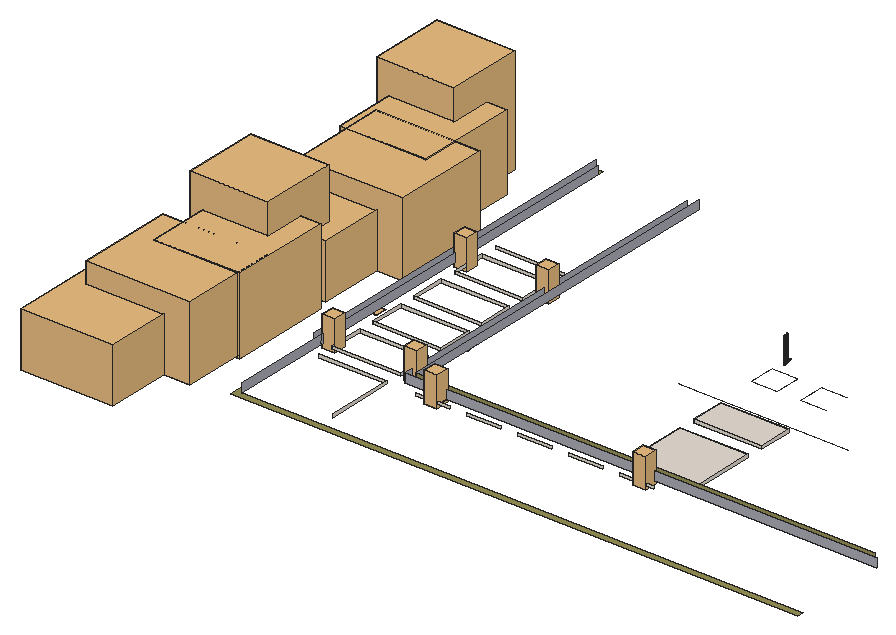
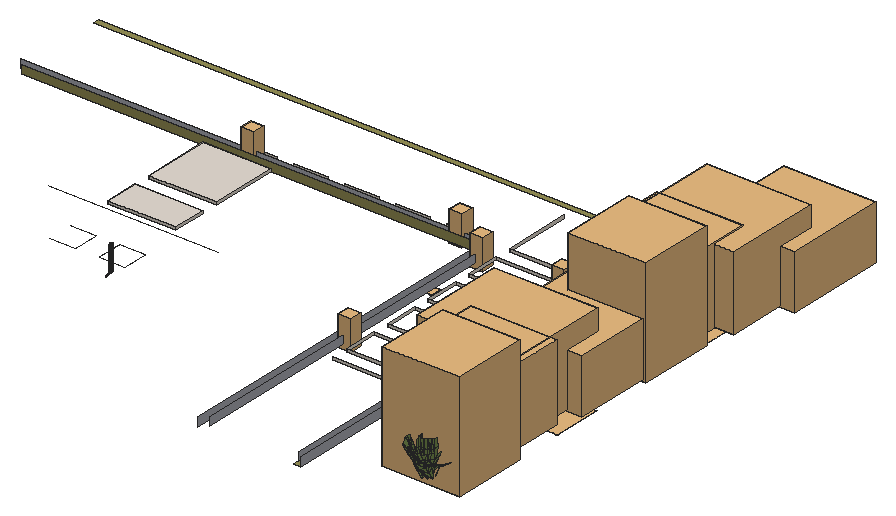
# SketchUp Ruby script. Lengths in inches.
U = 1.inch
M = Sketchup.active_model
def pt(a) = Geom::Point3d.new(a.map { |v| v * U })
def face(e, loops, mat)
  f = e.add_face(loops[0].map { |a| pt(a) })
  loops[1..].each { |l| e.add_face(l.map { |a| pt(a) }).erase! }
  f.material = f.back_material = mat if mat
  f
end
# faces: each face lists its corners as indices into pts; further lists are holes
def faces(e, pts, list, mat = nil) = list.each { |f| face(e, (f[0].is_a?(Array) ? f : [f]).map { |l| l.map { |i| pts[i] } }, mat) }
# xy, xz, yz: faces in a plane at the given z, y or x. An outline is a flat list of corners, or four numbers for a rectangle; further outlines are holes
def ring(l) = l.size == 4 ? [[l[0], l[1]], [l[2], l[1]], [l[2], l[3]], [l[0], l[3]]] : l.each_slice(2).to_a
def flat(e, list, mat, &to3) = list.each { |f| face(e, (f[0].is_a?(Array) ? f : [f]).map { |l| ring(l).map { |u, v| to3.(u, v) } }, mat) }
def xy(e, z, list, mat = nil) = flat(e, list, mat) { |x, y| [x, y, z] }
def xz(e, y, list, mat = nil) = flat(e, list, mat) { |x, z| [x, y, z] }
def yz(e, x, list, mat = nil) = flat(e, list, mat) { |y, z| [x, y, z] }
def lines(e, pts, list) = list.each { |a, b| e.add_line(pt(pts[a]), pt(pts[b])) }
# prism: a flat outline (further loops are holes) pulled along v
def prism(e, loops, v, mat = nil)
  f = face(e, loops, mat); d = Geom::Vector3d.new(v.map { |x| x * U })
  f.pushpull(f.normal.samedirection?(d) ? d.length : -d.length)
end
def box(e, o, s, mat = nil) = prism(e, [[o, [o[0] + s[0], o[1], o[2]], [o[0] + s[0], o[1] + s[1], o[2]], [o[0], o[1] + s[1], o[2]]]], [0, 0, s[2]], mat)
def at(x, y, z, deg = 0) = Geom::Transformation.translation(pt([x, y, z])) * Geom::Transformation.rotation(ORIGIN, Z_AXIS, deg.degrees)
def axes(o, x, y, z) = Geom::Transformation.new([*x, 0, *y, 0, *z, 0, *pt(o).to_a, 1])
def part(name) = M.definitions.add(name)
# library, detail: a bought-in or finely detailed component or shape, given as its bounding box
def library(name, o, s) = part(name).tap { |d| box(d.entities, o, s) }
def detail(e, o, s) = box(e.add_group.entities, o, s)
def put(e, d, t, mat = nil) = e.add_instance(d, t).tap { |i| i.material = mat if mat }
def group(e, t, mat = nil) = e.add_group.tap { |g| g.transformation = t; g.material = mat if mat }.entities
root = M.entities
M.materials.add("Marble_01_1K").color = [230, 221, 211]
M.materials.add("Marble_07_1K").color = [36, 34, 36]
M.materials.add("Marble_20_1K").color = [172, 173, 182]
M.materials.add("Material__4").color = [36, 36, 36]
M.materials.add("Material__6").color = [79, 108, 5]
M.materials.add("Plaster_06_1K").color = [141, 135, 122]
M.materials.add("Soil_04_1K").color = [152, 146, 88]
M.materials.add("calathea lutea").color = [121, 145, 80]
c1 = part("Group\#156")
g1 = group(c1.entities,at(8.61,38.85,0))
xy(g1,0,[[0,0,2.82,19.1,22.58,0],[22.58,0,2.82,19.1,22.58,19.1]],"calathea lutea")
p = [[2.82,19.1,0],[7.19,48.22,5.13],[10.77,48.22,5.13],[12.74,48.22,5.13],[22.58,48.22,5.13],[22.58,19.1,0]]
faces(g1,p,[[0,1,2,3,4,5]],"calathea lutea")
g2 = group(c1.entities,at(-0.77,-7.77,0))
p = [[14.8125,23.31,1.46],[21.35,23.31,0],[14.8125,0,1.46],[21.35,0,0],[27.89,0,1.46],[27.89,23.31,1.46],
  [8.27,46.62,2.92],[21.35,46.62,0],[34.4375,46.62,2.92],[4.47,23.31,6.43],[0,0,8.59],[33.76,0,4.28],
  [33.76,23.31,4.28]]
faces(g2,p,[[0,1,2],[3,2,1],[4,3,5],[1,5,3],[6,7,0],[1,0,7],[5,1,8],[7,8,1],
  [9,0,2,10],[11,4,5,12],[9,6,0],[12,5,8]],"calathea lutea")
c2 = part("Group\#150")
xy(c2.entities,0,[[0,0,0,33.87,27.21,33.87,19.71,0]],"calathea lutea")
c3 = part("Group\#157")
xy(c3.entities,1.04,[[21.13,33.87,21.13,57.59,32.375,57.59,27.12,33.87]],"calathea lutea")
xy(c3.entities,1.32,[[0.12,33.87,7.74,57.59]],"calathea lutea")
p = [[7.74,33.87,1.32],[11.8,57.59,0.61],[15.24,57.59,0],[15.24,33.87,0],[18.43,57.59,0.5625],[21.13,57.59,1.04],
  [21.13,33.87,1.04],[15.24,77.7,2.36],[21.13,77.7,3.4],[7.74,57.59,1.32],[7.74,77.7,3.69],[36.83,77.7,3.4],
  [32.375,57.59,1.04],[0.12,57.59,1.32],[0.12,77.7,3.69]]
faces(c3.entities,p,[[0,1,2,3],[3,2,4],[3,4,5,6],[7,2,1],[8,4,2,7],[0,9,1],[7,1,9,10],[8,5,4],
  [11,12,5,8],[10,9,13,14]],"calathea lutea")
put(c3.entities,c2,axes([0,-16.9375,0],[1,0,0],[0,1.5,0],[0,0,1]))
c4 = part("Group\#155")
g3 = group(c4.entities,at(0,-17.3,0))
xy(g3,0,[[0,0,28.07,51.9]],"calathea lutea")
g4 = group(c4.entities,at(0.9,34.6,0))
xy(g4,0,[[13.14,0,13.14,26.22,16.85,26.22],[13.14,0,16.85,26.22,20.16,26.22,20.16,0]],"calathea lutea")
p = [[6.36,0,1.82],[9.95,26.22,0.86],[13.14,26.22,0],[13.14,0,0],[20.16,0,0],[20.16,26.22,0],
  [27.07,26.22,1.22],[27.07,0,1.22],[13.14,49.5625,5.91],[20.16,49.5625,5.91],[16.85,26.22,0],[27.07,49.5625,7.125],
  [6.36,26.22,1.82],[6.36,49.5625,7.72],[0,0,4.78],[0,26.22,4.78],[0,49.5625,10.6875]]
faces(g4,p,[[0,1,2,3],[4,5,6,7],[8,2,1],[9,10,2,8],[9,5,10],[11,6,5,9],[0,12,1],[8,1,12,13],
  [14,15,12,0],[13,12,15,16]],"calathea lutea")
c5 = part("Group\#154")
put(c5.entities,c2,axes([0,-16.9375,0],[1,0,0],[0,1.5,0],[0,0,1]))
g5 = group(c5.entities,at(-0.23,33.4,-0.35))
p = [[15.12,39.14,-19.87],[15.12,20.54,-11.86],[11.68,20.84,-11.33],[21.02,39.66,-18.97],[18.3125,20.82,-11.37],[7.62,21.2,-10.71],
  [7.62,39.8,-18.72],[21.02,21.06,-10.96],[36.72,39.66,-18.97],[32.26,21.06,-10.96],[0,21.2,-10.71],[0,39.8,-18.72],
  [7.62,0.66,1.15],[15.12,0,0],[21.02,0.52,0.9],[27.01,0.52,0.9],[0,0.66,1.15]]
faces(g5,p,[[0,1,2],[3,4,1,0],[0,2,5,6],[3,7,4],[8,9,7,3],[6,5,10,11],[12,2,1,13],[13,1,4],
  [13,4,7,14],[12,5,2],[14,7,9,15],[16,10,5,12]],"calathea lutea")
c6 = part("Foliage cluster")
put(c6.entities,c1,axes([37.24,8.07,75.17],[1,0,0],[0,0.45554,-0.89021],[0,0.89021,0.45554]))
put(c6.entities,c3,axes([69.44,65.48,16.68],[-0.53288,-0.84619,0],[0.14694,-0.09253,0.98481],[-0.83334,0.52478,0.17365]))
put(c6.entities,c4,axes([47.9375,70.43,17.04],[0.74664,-0.66523,0],[0.11552,0.12965,0.98481],[-0.65512,-0.7353,0.17365]))
put(c6.entities,c1,axes([76.19,10.66,75.17],[0.70711,0.70711,0],[-0.32212,0.32212,-0.89021],[-0.62948,0.62948,0.45554]))
put(c6.entities,c1,axes([101.91,40.03,75.17],[0,1,0],[-0.45554,0,-0.89021],[-0.89021,0,0.45554]))
put(c6.entities,c1,axes([99.32,78.99,75.17],[-0.70711,0.70711,0],[-0.32212,-0.32212,-0.89021],[-0.62948,-0.62948,0.45554]))
put(c6.entities,c4,axes([34.81,63.36,17.04],[0.99956,-0.02967,0],[0.00515,0.17357,0.98481],[-0.02922,-0.98437,0.17365]))
put(c6.entities,c4,axes([48,37.4,15.8],[-0.14436,0.98953,0],[-0.40248,-0.05871,0.91355],[0.90398,0.13188,0.40674]))
put(c6.entities,c3,axes([56.87,39.77,12.28],[-0.67695,0.4263,0],[-0.18016,-0.28609,0.72505],[0.38636,0.61353,0.33809]))
put(c6.entities,c3,axes([36.12,43.25,12.28],[0.18947,0.77724,0],[-0.32848,0.08007,0.72505],[0.70442,-0.17172,0.33809]))
put(c6.entities,c5,axes([35.1,54.93,11.375],[0.79719,0.06694,0],[-0.03636,0.43302,0.6717],[0.05621,-0.66934,0.43454]))
put(c6.entities,c3,axes([41.66,47.32,12.28],[0.45082,0.66088,0],[-0.2793,0.19053,0.72505],[0.59896,-0.40858,0.33809]))
put(c6.entities,c3,axes([47.89,59.4,12.28],[0.79719,0.06694,0],[-0.02829,0.33691,0.72505],[0.06067,-0.7225,0.33809]))
put(c6.entities,c5,axes([29.53,49.96,11.375],[0.65692,0.45657,0],[-0.248,0.35682,0.6717],[0.38335,-0.55156,0.43454]))
put(c6.entities,c5,axes([29.9,49.27,12.86],[0.34062,0.72386,0],[-0.22849,0.10752,0.7591],[0.68685,-0.32321,0.25252]))
put(c6.entities,c5,axes([36.33,48.82,8.99],[0.09232,0.62522,0],[-0.3396,0.05015,0.53064],[0.52495,-0.07752,0.34329]))
put(c6.entities,c5,axes([49.82,38.52,8.99],[-0.54622,0.31791,0],[-0.17268,-0.29669,0.53064],[0.26692,0.45862,0.34329]))
put(c6.entities,c5,axes([55.68,39.21,8.99],[-0.632,0.00221,0],[-0.0012,-0.34328,0.53064],[0.00185,0.53064,0.34329]))
c7 = library("Group\#28",[0,0,0],[86.94,78.77,46.4375])
c8 = library("Group\#14",[-978.71,-103.24,719.12],[90.2,76.4,68.29])
c9 = library("Group\#13",[-906.16,-138.28,686.8],[98.25,106.18,75.79])
c10 = library("Group\#202",[-3.47,-2.45,12.47],[53.14,54.93,75.51])
c11 = part("Group\#41")
put(c11.entities,c6,axes([161.54,64.35,6.01],[0.19523,-0.19694,0],[0.19694,0.19523,0],[0,0,0.24957]))
put(c11.entities,c7,axes([0,37.34,0.92],[0.83,0,0],[0,0.83,0],[0,0,0.83]))
put(c11.entities,c8,axes([859.63,98.87,-568.1],[0.79,0,0],[0,0.79,0],[0,0,0.79]),"Material__4")
put(c11.entities,c9,axes([669.69,114.28,-472.48],[0.69,0,0],[0,0.69,0],[0,0,0.69]),"Material__6")
put(c11.entities,c10,at(132.78,33.9375,-12.6))
c12 = library("Group\#54",[0,0,0],[2062.46,2062.46,4833.66])
c13 = part("Landscape+Light")
put(c13.entities,c12,at(-2096.57,-1031.23,-3775.98))
c14 = library("light",[-4,-4,0],[8,8,0.01])
c15 = library("t1",[-17.79,-17.21,0],[35.58,34.42,0.01])
c16 = library("tt",[-12.4,-12.1,0],[24.8,24.2,0.01])
c17 = library("ew",[-14.92,-16.84,0],[29.84,33.68,0.01])
c18 = part("Group\#40")
put(c18.entities,c6,axes([161.54,64.35,6.01],[0.19523,-0.19694,0],[0.19694,0.19523,0],[0,0,0.24957]))
put(c18.entities,c7,axes([0,18.48,0.92],[0.83,0,0],[0,0.83,0],[0,0,0.83]))
put(c18.entities,c8,axes([859.63,98.87,-568.1],[0.79,0,0],[0,0.79,0],[0,0,0.79]),"Material__4")
put(c18.entities,c9,axes([669.69,95.42,-472.48],[0.69,0,0],[0,0.69,0],[0,0,0.69]),"Material__6")
put(c18.entities,c10,at(132.78,33.9375,-12.6))
box(root,[318.11,636.64,0],[48,48,2],"Marble_01_1K")
box(root,[318.11,696.64,0],[48,24,2],"Marble_01_1K")
xy(root,0,[[317.04,778.3125,317.09,778.3125,317.07,778.39,317.05,778.44,317,778.52,316.99,778.56,316.97,778.6,316.95,778.66,316.93,778.71,316.91,778.81,316.92,778.86,316.92,778.91,316.93,778.96,316.97,779.06,317,779.11,317.02,779.16,317.06,779.22,317.08,779.27,317.17,779.42,317.19,779.47,317.2,779.53,317.21,779.58,317.19,779.65,317.18,779.69,317.16,779.76,317.15,779.8,317.11,779.84,317.07,779.92,317.05,779.95,316.99,780.03,316.94,780.1,316.91,780.16,316.875,780.1875,316.84,780.24,316.82,780.28,316.79,780.33,316.73,780.41,316.74,780.47,316.75,780.51,316.75,780.56,316.76,780.6,316.76,780.7,316.78,780.74,316.78,780.8,316.79,780.86,316.79,780.98,316.78,781.02,316.78,781.07,316.76,781.125,316.75,781.17,316.74,781.21,316.73,781.26,316.71,781.32,316.7,781.36,316.69,781.41,316.67,781.47,316.65,781.51,316.65,781.56,316.58,781.7,316.55,781.74,316.52,781.79,316.51,781.85,316.5,781.9,316.51,781.95,316.57,782.1,316.61,782.18,316.65,782.22,316.67,782.26,316.7,782.3,316.7,782.41,316.66,782.51,316.6,782.61,316.57,782.64,316.52,782.7,316.49,782.73,316.45,782.76,316.41,782.82,316.35,782.88,316.3,782.94,316.27,782.99,316.25,783.02,316.21,783.06,316.15,783.15,316.13,783.19,316.1,783.24,316.1,783.29,316.09,783.33,316.07,783.42,316.07,783.46,316.08,783.51,316.08,783.65,316.09,783.71,316.1,783.75,316.12,783.79,316.13,783.84,316.125,783.89,316.14,783.93,316.14,784.04,316.13,784.08,316.13,784.13,316.125,784.17,316.12,784.22,316.1,784.27,316.08,784.31,316.06,784.36,316.05,784.4,316.02,784.4375,316,784.49,315.97,784.53,315.9375,784.57,315.91,784.62,315.85,784.7,315.83,784.75,315.8,784.79,315.78,784.83,315.76,784.875,315.75,784.92,315.75,784.97,315.73,785.02,315.72,785.06,315.7,785.1,315.69,785.15,315.67,785.19,315.64,785.24,315.62,785.29,315.49,785.42,315.45,785.45,315.42,785.48,315.26,785.53,315.24,785.44,315.27,785.32,315.28,785.29,315.28,785.23,315.29,785.19,315.29,785.15,315.31,785.11,315.32,785.05,315.33,785.01,315.35,784.96,315.36,784.9,315.39,784.86,315.4,784.8125,315.41,784.76,315.4375,784.71,315.45,784.67,315.46,784.63,315.46,784.59,315.48,784.55,315.49,784.51,315.51,784.46,315.52,784.41,315.52,784.37,315.54,784.33,315.54,784.29,315.55,784.23,315.55,784.07,315.54,784.02,315.54,783.91,315.53,783.87,315.54,783.81,315.53,783.75,315.53,783.7,315.55,783.6,315.59,783.5,315.6,783.46,315.61,783.4,315.64,783.35,315.66,783.29,315.68,783.26,315.68,783.21,315.71,783.15,315.75,783.05,315.76,783.01,315.8,782.91,315.82,782.87,315.83,782.82,315.86,782.78,315.88,782.73,315.9,782.6875,315.91,782.65,315.93,782.6,315.94,782.52,315.9375,782.48,315.93,782.4375,315.93,782.39,315.91,782.35,315.9,782.29,315.88,782.23,315.88,782.1875,315.87,782.125,315.86,782.06,315.84,781.98,315.85,781.92,315.86,781.87,315.86,781.8125,315.88,781.76,315.91,781.7,315.93,781.65,315.99,781.55,316.01,781.49,316.04,781.4375,316.07,781.39,316.1,781.34,316.125,781.3,316.16,781.26,316.18,781.21,316.21,781.17,316.23,781.11,316.26,781.06,316.3,781.02,316.33,780.97,316.36,780.93,316.42,780.83,316.44,780.79,316.42,780.72,316.41,780.68,316.39,780.63,316.375,780.59,316.35,780.53,316.32,780.49,316.3,780.44,316.28,780.4,316.27,780.35,316.25,780.31,316.23,780.26,316.22,780.21,316.21,780.15,316.21,780.1,316.22,780.03,316.23,779.98,316.22,779.93,316.23,779.86,316.24,779.8125,316.23,779.75,316.26,779.66,316.26,779.62,316.27,779.58,316.29,779.52,316.3125,779.45,316.33,779.41,316.36,779.33,316.39,779.3,316.4,779.25,316.46,779.13,316.47,779.08,316.49,779.03,316.48,778.99,316.49,778.9375,316.48,778.89,316.46,778.85,316.43,778.78,316.39,778.7,316.36,778.65,316.34,778.61,316.32,778.5625,316.3125,778.52,316.35,778.48,316.41,778.43,316.47,778.42,316.57,778.4,316.65,778.38,316.75,778.37,316.93,778.33,316.99,778.32]],"Marble_07_1K")
xy(root,0,[[98.71,562.78,98.71,885.25,103.21,885.25,103.21,567.28,498.69,567.28,498.69,562.78]],"Soil_04_1K")
xz(root,624.64,[[111.43,0,159.43,2],[180.08,0,204.08,2],[216.08,0,240.08,2],[252.08,0,276.08,2],[288.08,0,312.08,2],
  [324.08,0,348.08,2]],"Marble_01_1K")
xz(root,632.1,[[166.21,0,498.69,6]],"Marble_20_1K")
xz(root,636.6,[[170.71,0,494.19,6]],"Soil_04_1K")
xz(root,636.64,[[111.43,0,159.43,2]],"Marble_01_1K")
xz(root,660.64,[[111.43,0,159.43,2]],"Marble_01_1K")
xz(root,672.64,[[111.43,0,159.43,2]],"Marble_01_1K")
xz(root,696.64,[[111.43,0,159.43,2]],"Marble_01_1K")
xz(root,708.64,[[111.43,0,159.43,2]],"Marble_01_1K")
xz(root,732.64,[[111.43,0,159.43,2]],"Marble_01_1K")
xz(root,744.64,[[111.43,0,159.43,2]],"Marble_01_1K")
xz(root,768.64,[[111.43,0,159.43,2]],"Marble_01_1K")
xz(root,778.3125,[[317.04,0,317.09,18]],"Marble_07_1K")
xz(root,780.64,[[111.43,0,159.43,2]],"Marble_01_1K")
yz(root,98.71,[[636.6,0,885.25,6]],"Marble_20_1K")
yz(root,103.21,[[567.28,0,636.6,6],[636.6,0,880.75,6]],"Marble_20_1K")
yz(root,111.43,[[636.64,0,660.64,2],[672.64,0,696.64,2],[708.64,0,732.64,2],[744.64,0,768.64,2]],"Marble_01_1K")
yz(root,159.43,[[576.78,0,624.64,2],[636.64,0,660.64,2],[672.64,0,696.64,2],[708.64,0,732.64,2],[744.64,0,768.64,2]],"Marble_01_1K")
yz(root,166.21,[[632.1,0,880.75,6]],"Marble_20_1K")
yz(root,170.71,[[636.6,0,885.25,6]],"Marble_20_1K")
yz(root,315.86,[[781.8125,0,781.87,18]],"Marble_07_1K")
yz(root,316.21,[[780.1,0,780.15,18]],"Marble_07_1K")
yz(root,316.26,[[779.62,0,779.66,18]],"Marble_07_1K")
yz(root,316.65,[[781.51,0,781.56,18]],"Marble_07_1K")
yz(root,316.75,[[780.51,0,780.56,18]],"Marble_07_1K")
yz(root,316.76,[[780.6,0,780.65,18],[780.65,0,780.7,18]],"Marble_07_1K")
yz(root,316.78,[[780.74,0,780.8,18],[781.02,0,781.07,18]],"Marble_07_1K")
yz(root,316.79,[[780.86,0,780.92,18],[780.92,0,780.98,18]],"Marble_07_1K")
yz(root,316.92,[[778.86,0,778.91,18]],"Marble_07_1K")
p = [[49.91,608.6,0],[48.07,599.64,0],[48.07,599.64,6],[49.91,608.6,6],[51.66,602.1875,0],[53.72,612.24,0],
  [53.72,612.24,6],[51.66,602.1875,6],[51.74,617.54,0],[51.74,617.54,6],[55.76,622.29,0],[55.76,622.29,6],
  [53.52,626.45,0],[53.52,626.45,6],[57.72,632.32,0],[57.72,632.32,6],[55.24,635.36,0],[55.24,635.36,6],
  [59.56,642.35,0],[59.56,642.35,6],[56.85,644.25,0],[56.85,644.25,6],[61.25,652.38,0],[61.25,652.38,6],
  [58.34,653.13,0],[58.34,653.13,6],[62.74,662.42,0],[62.74,662.42,6],[59.66,662.01,0],[59.66,662.01,6],
  [60.79,670.88,0],[60.79,670.88,6],[63.99,672.47,0],[63.99,672.47,6],[61.71,679.76,0],[61.71,679.76,6],
  [64.95,682.54,0],[64.95,682.54,6],[62.39,688.65,0],[62.39,688.65,6],[65.62,692.62,0],[65.62,692.62,6],
  [62.84,697.5625,0],[62.84,697.5625,6],[66,702.73,0],[66,702.73,6],[63.07,706.49,0],[63.07,706.49,6],
  [66.125,712.84,0],[66.125,712.84,6],[63.12,715.44,0],[63.12,715.44,6],[66.01,722.98,0],[66.01,722.98,6],
  [62.98,724.4,0],[62.98,724.4,6],[65.68,733.125,0],[65.68,733.125,6],[62.67,733.375,0],[62.67,733.375,6],
  [65.16,743.28,0],[65.16,743.28,6],[62.21,742.37,0],[62.21,742.37,6],[61.61,751.38,0],[61.61,751.38,6],
  [64.47,753.45,0],[64.47,753.45,6],[60.89,760.4,0],[60.89,760.4,6],[63.62,763.63,0],[63.62,763.63,6],
  [60.07,769.43,0],[60.07,769.43,6],[62.65,773.82,0],[62.65,773.82,6],[59.15,778.47,0],[59.15,778.47,6],
  [61.57,784.01,0],[61.57,784.01,6],[316.84,778.35,0],[316.84,778.35,18],[316.93,778.33,18],[316.93,778.33,0],
  [316.99,778.32,18],[316.99,778.32,0],[317.04,778.3125,18],[317.04,778.3125,0],[317.09,778.3125,0],[317.09,778.3125,18],
  [317.07,778.39,18],[317.07,778.39,0],[316.41,778.43,0],[316.41,778.43,18],[316.47,778.42,18],[316.47,778.42,0],
  [316.35,778.48,0],[316.35,778.48,18],[316.57,778.4,18],[316.57,778.4,0],[316.65,778.38,18],[316.65,778.38,0],
  [316.75,778.37,0],[316.75,778.37,18],[317.05,778.44,0],[317.05,778.44,18],[317,778.52,18],[317,778.52,0],
  [316.3125,778.52,0],[316.3125,778.52,18],[316.32,778.5625,0],[316.32,778.5625,18],[316.99,778.56,18],[316.99,778.56,0],
  [316.34,778.61,0],[316.34,778.61,18],[316.36,778.65,0],[316.36,778.65,18],[316.97,778.6,0],[316.97,778.6,18],
  [316.95,778.66,18],[316.95,778.66,0],[316.39,778.7,0],[316.39,778.7,18],[316.41,778.74,0],[316.41,778.74,18],
  [316.43,778.78,0],[316.43,778.78,18],[316.93,778.71,18],[316.93,778.71,0],[316.92,778.76,18],[316.92,778.76,0],
  [316.46,778.85,0],[316.46,778.85,18],[316.48,778.89,0],[316.48,778.89,18],[316.91,778.81,18],[316.91,778.81,0],
  [316.92,778.86,18],[316.92,778.86,0],[316.49,778.9375,0],[316.49,778.9375,18],[316.48,778.99,0],[316.48,778.99,18],
  [316.92,778.91,0],[316.92,778.91,18],[316.93,778.96,18],[316.93,778.96,0],[316.49,779.03,0],[316.49,779.03,18],
  [316.47,779.08,0],[316.47,779.08,18],[316.95,779.01,18],[316.95,779.01,0],[316.97,779.06,18],[316.97,779.06,0],
  [316.43,779.19,0],[316.43,779.19,18],[316.46,779.13,18],[316.46,779.13,0],[317,779.11,18],[317,779.11,0],
  [317.02,779.16,18],[317.02,779.16,0],[316.4,779.25,0],[316.4,779.25,18],[316.39,779.3,0],[316.39,779.3,18],
  [317.06,779.22,18],[317.06,779.22,0],[317.08,779.27,18],[317.08,779.27,0],[316.33,779.41,0],[316.33,779.41,18],
  [316.36,779.33,18],[316.36,779.33,0],[317.11,779.32,18],[317.11,779.32,0],[317.14,779.37,18],[317.14,779.37,0],
  [316.3125,779.45,0],[316.3125,779.45,18],[317.17,779.42,18],[317.17,779.42,0],[317.19,779.47,18],[317.19,779.47,0],
  [316.29,779.52,0],[316.29,779.52,18],[316.27,779.58,0],[316.27,779.58,18],[317.2,779.53,18],[317.2,779.53,0],
  [317.21,779.58,18],[317.21,779.58,0],[316.26,779.62,0],[316.26,779.62,18],[317.19,779.65,18],[317.19,779.65,0],
  [317.18,779.69,18],[317.18,779.69,0],[316.23,779.75,0],[316.23,779.75,18],[316.26,779.66,18],[316.26,779.66,0],
  [316.24,779.8125,0],[316.24,779.8125,18],[317.16,779.76,18],[317.16,779.76,0],[316.23,779.86,0],[316.23,779.86,18],
  [317.15,779.8,18],[317.15,779.8,0],[317.11,779.84,18],[317.11,779.84,0],[317.07,779.92,18],[317.07,779.92,0],
  [316.22,779.93,0],[316.22,779.93,18],[316.23,779.98,0],[316.23,779.98,18],[317.05,779.95,18],[317.05,779.95,0],
  [316.22,780.03,0],[316.22,780.03,18],[316.21,780.1,0],[316.21,780.1,18],[316.99,780.03,0],[316.99,780.03,18],
  [316.94,780.1,18],[316.94,780.1,0],[317.02,779.99,18],[317.02,779.99,0],[316.91,780.16,18],[316.91,780.16,0],
  [316.22,780.21,0],[316.22,780.21,18],[316.21,780.15,18],[316.21,780.15,0],[316.23,780.26,0],[316.23,780.26,18],
  [316.875,780.1875,0],[316.875,780.1875,18],[316.84,780.24,18],[316.84,780.24,0],[316.82,780.28,18],[316.82,780.28,0],
  [316.25,780.31,0],[316.25,780.31,18],[316.27,780.35,0],[316.27,780.35,18],[316.79,780.33,18],[316.79,780.33,0],
  [316.76,780.37,18],[316.76,780.37,0],[316.28,780.4,0],[316.28,780.4,18],[316.3,780.44,0],[316.3,780.44,18],
  [316.32,780.49,0],[316.32,780.49,18],[316.73,780.41,18],[316.73,780.41,0],[316.74,780.47,18],[316.74,780.47,0],
  [316.35,780.53,0],[316.35,780.53,18],[316.375,780.59,0],[316.375,780.59,18],[316.75,780.51,18],[316.75,780.51,0],
  [316.39,780.63,0],[316.39,780.63,18],[316.41,780.68,0],[316.41,780.68,18],[316.75,780.56,0],[316.75,780.56,18],
  [316.76,780.6,18],[316.76,780.6,0],[316.42,780.72,0],[316.42,780.72,18],[316.44,780.79,0],[316.44,780.79,18],
  [316.76,780.7,0],[316.76,780.7,18],[316.78,780.74,18],[316.78,780.74,0],[316.42,780.83,0],[316.42,780.83,18],
  [316.39,780.88,0],[316.39,780.88,18],[316.78,780.8,0],[316.78,780.8,18],[316.79,780.86,18],[316.79,780.86,0],
  [316.33,780.97,0],[316.33,780.97,18],[316.36,780.93,18],[316.36,780.93,0],[316.3,781.02,0],[316.3,781.02,18],
  [316.26,781.06,0],[316.26,781.06,18],[316.79,780.98,0],[316.79,780.98,18],[316.78,781.02,18],[316.78,781.02,0],
  [316.23,781.11,0],[316.23,781.11,18],[316.21,781.17,0],[316.21,781.17,18],[316.76,781.125,0],[316.76,781.125,18],
  [316.75,781.17,18],[316.75,781.17,0],[316.78,781.07,0],[316.78,781.07,18],[316.18,781.21,0],[316.18,781.21,18],
  [316.16,781.26,0],[316.16,781.26,18],[316.74,781.21,18],[316.74,781.21,0],[316.73,781.26,18],[316.73,781.26,0],
  [316.125,781.3,0],[316.125,781.3,18],[316.1,781.34,0],[316.1,781.34,18],[316.07,781.39,0],[316.07,781.39,18],
  [316.71,781.32,18],[316.71,781.32,0],[316.7,781.36,18],[316.7,781.36,0],[316.04,781.4375,0],[316.04,781.4375,18],
  [316.01,781.49,0],[316.01,781.49,18],[316.69,781.41,18],[316.69,781.41,0],[316.67,781.47,18],[316.67,781.47,0],
  [315.99,781.55,0],[315.99,781.55,18],[315.96,781.6,0],[315.96,781.6,18],[316.65,781.51,18],[316.65,781.51,0],
  [315.93,781.65,0],[315.93,781.65,18],[316.65,781.56,0],[316.65,781.56,18],[316.625,781.61,18],[316.625,781.61,0],
  [316.6,781.66,18],[316.6,781.66,0],[315.91,781.7,0],[315.91,781.7,18],[315.88,781.76,0],[315.88,781.76,18],
  [316.58,781.7,0],[316.58,781.7,18],[316.55,781.74,18],[316.55,781.74,0],[316.52,781.79,18],[316.52,781.79,0],
  [315.86,781.8125,0],[315.86,781.8125,18],[316.51,781.85,18],[316.51,781.85,0],[316.5,781.9,18],[316.5,781.9,0],
  [315.84,781.98,0],[315.84,781.98,18],[315.85,781.92,18],[315.85,781.92,0],[315.86,781.87,18],[315.86,781.87,0],
  [316.51,781.95,18],[316.51,781.95,0],[316.53,782,18],[316.53,782,0],[404.37,725.46,0],[284.28,725.46,0],
  [332.34,752.53,0],[332.34,754.74,0],[332.34,770.83,0],[314.04,770.83,0],[314.04,752.53,0],[332.36,754.74,0],
  [366.875,771.18,0],[348.57,771.18,0],[348.57,752.88,0],[366.875,752.88,0]]
faces(root,p,[[0,1,2,3],[8,0,3,9],[12,8,9,13],[16,12,13,17],[20,16,17,21],[24,20,21,25],[28,24,25,29],[30,28,29,31],
  [34,30,31,35],[38,34,35,39],[42,38,39,43],[46,42,43,47],[50,46,47,51],[54,50,51,55],[58,54,55,59],[62,58,59,63],
  [64,62,63,65],[68,64,65,69],[72,68,69,73],[76,72,73,77]])
faces(root,p,[[4,5,6,7],[5,10,11,6],[10,14,15,11],[14,18,19,15],[18,22,23,19],[22,26,27,23],[26,32,33,27],[32,36,37,33],
  [36,40,41,37],[40,44,45,41],[44,48,49,45],[48,52,53,49],[52,56,57,53],[56,60,61,57],[60,66,67,61],[66,70,71,67],
  [70,74,75,71],[74,78,79,75]],"Plaster_06_1K")
faces(root,p,[[80,81,82,83],[83,82,84,85],[85,84,86,87],[88,89,90,91],[92,93,94,95],[96,97,93,92],[95,94,98,99],[99,98,100,101],
  [102,103,81,80],[101,100,103,102],[104,105,106,107],[91,90,105,104],[108,109,97,96],[110,111,109,108],[107,106,112,113],[114,115,111,110],
  [116,117,115,114],[118,119,120,121],[113,112,119,118],[122,123,117,116],[124,125,123,122],[126,127,125,124],[121,120,128,129],[129,128,130,131],
  [132,133,127,126],[134,135,133,132],[131,130,136,137],[137,136,138,139],[140,141,135,134],[142,143,141,140],[144,145,146,147],[148,149,143,142],
  [150,151,149,148],[147,146,152,153],[153,152,154,155],[156,157,158,159],[159,158,151,150],[155,154,160,161],[161,160,162,163],[164,165,157,156],
  [166,167,165,164],[163,162,168,169],[169,168,170,171],[172,173,174,175],[175,174,167,166],[171,170,176,177],[177,176,178,179],[180,181,173,172],
  [179,178,182,183],[183,182,184,185],[186,187,181,180],[188,189,187,186],[185,184,190,191],[191,190,192,193],[194,195,189,188],[193,192,196,197],
  [197,196,198,199],[200,201,202,203],[204,205,201,200],[199,198,206,207],[208,209,205,204],[207,206,210,211],[211,210,212,213],[213,212,214,215],
  [216,217,209,208],[218,219,217,216],[215,214,220,221],[222,223,219,218],[224,225,223,222],[226,227,228,229],[221,220,230,231],[231,230,227,226],
  [229,228,232,233],[234,235,236,237],[238,239,235,234],[240,241,242,243],[243,242,244,245],[233,232,241,240],[246,247,239,238],[248,249,247,246],
  [245,244,250,251],[251,250,252,253],[254,255,249,248],[256,257,255,254],[258,259,257,256],[253,252,260,261],[261,260,262,263],[264,265,259,258],
  [266,267,265,264],[263,262,268,269],[270,271,267,266],[272,273,271,270],[274,275,276,277],[278,279,273,272],[280,281,279,278],[282,283,284,285],
  [286,287,281,280],[288,289,287,286],[290,291,292,293],[294,295,296,297],[297,296,289,288],[298,299,295,294],[300,301,299,298],[302,303,304,305],
  [306,307,301,300],[308,309,307,306],[310,311,312,313],[314,315,311,310],[316,317,309,308],[318,319,317,316],[313,312,320,321],[321,320,322,323],
  [324,325,319,318],[326,327,325,324],[328,329,327,326],[323,322,330,331],[331,330,332,333],[334,335,329,328],[336,337,335,334],[333,332,338,339],
  [339,338,340,341],[342,343,337,336],[344,345,343,342],[341,340,346,347],[348,349,345,344],[350,351,352,353],[353,352,354,355],[356,357,349,348],
  [358,359,357,356],[360,361,362,363],[363,362,364,365],[355,354,361,360],[366,367,359,358],[365,364,368,369],[369,368,370,371],[372,373,374,375],
  [375,374,376,377],[371,370,378,379],[379,378,380,381]],"Marble_07_1K")
lines(root,p,[[382,383],[384,385],[386,387],[387,388],[388,384],[385,389],[390,391],[391,392],[392,393],[385,386]])
put(root,c11,at(95.48,509.99,0.12,90))
put(root,c13,axes([185.79,629.125,13.79],[-0.0044,0,0],[0,-0.0044,0],[0,0,0.0044]))
put(root,c13,axes([332.82,629.125,13.79],[-0.0044,0,0],[0,-0.0044,0],[0,0,0.0044]))
put(root,c14,at(192.08,632.3,0))
put(root,c15,at(28.39,636.14,0,180))
put(root,c13,axes([107.4,647.56,13.79],[0,0.0044,0],[-0.0044,0,0],[0,0,0.0044]))
put(root,c13,axes([164.91,647.56,13.79],[0,0.0044,0],[-0.0044,0,0],[0,0,0.0044]))
put(root,c16,at(28.88,670.65,0,180))
put(root,c14,at(102.85,685.79,0,-90))
put(root,c14,at(166.71,685.79,0,-90))
put(root,c17,at(30.54,707.09,0,180))
put(root,c15,at(28.39,751.33,0,180))
put(root,c13,axes([107.4,763.92,13.79],[0,0.0044,0],[-0.0044,0,0],[0,0,0.0044]))
put(root,c13,axes([164.91,763.92,13.79],[0,0.0044,0],[-0.0044,0,0],[0,0,0.0044]))
put(root,c18,at(95.48,674.14,0.12,90))
